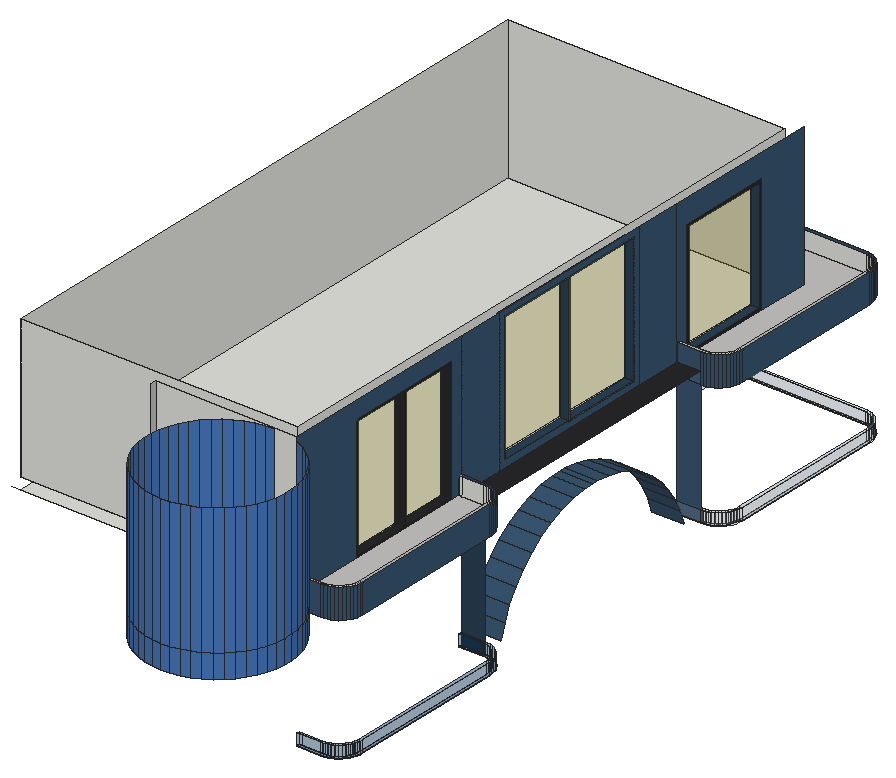
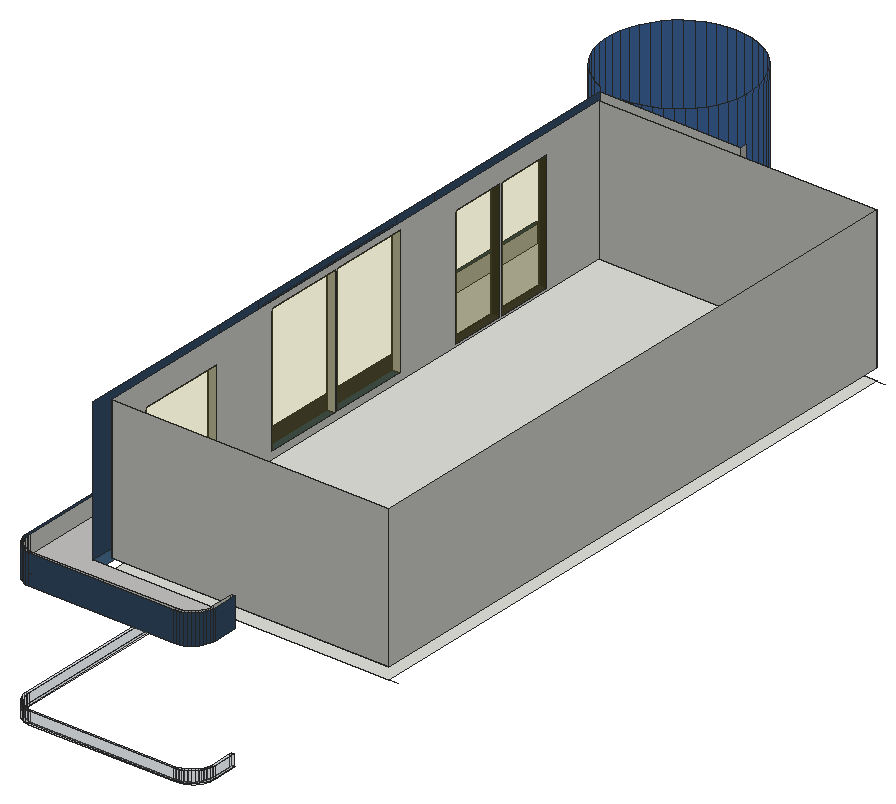
# SketchUp Ruby script. Lengths in inches.
U = 1.inch
M = Sketchup.active_model
def pt(a) = Geom::Point3d.new(a.map { |v| v * U })
def face(e, loops, mat)
  f = e.add_face(loops[0].map { |a| pt(a) })
  loops[1..].each { |l| e.add_face(l.map { |a| pt(a) }).erase! }
  f.material = f.back_material = mat if mat
  f
end
# faces: each face lists its corners as indices into pts; further lists are holes
def faces(e, pts, list, mat = nil) = list.each { |f| face(e, (f[0].is_a?(Array) ? f : [f]).map { |l| l.map { |i| pts[i] } }, mat) }
# xy, xz, yz: faces in a plane at the given z, y or x. An outline is a flat list of corners, or four numbers for a rectangle; further outlines are holes
def ring(l) = l.size == 4 ? [[l[0], l[1]], [l[2], l[1]], [l[2], l[3]], [l[0], l[3]]] : l.each_slice(2).to_a
def flat(e, list, mat, &to3) = list.each { |f| face(e, (f[0].is_a?(Array) ? f : [f]).map { |l| ring(l).map { |u, v| to3.(u, v) } }, mat) }
def xy(e, z, list, mat = nil) = flat(e, list, mat) { |x, y| [x, y, z] }
def xz(e, y, list, mat = nil) = flat(e, list, mat) { |x, z| [x, y, z] }
def yz(e, x, list, mat = nil) = flat(e, list, mat) { |y, z| [x, y, z] }
def lines(e, pts, list) = list.each { |a, b| e.add_line(pt(pts[a]), pt(pts[b])) }
# prism: a flat outline (further loops are holes) pulled along v
def prism(e, loops, v, mat = nil)
  f = face(e, loops, mat); d = Geom::Vector3d.new(v.map { |x| x * U })
  f.pushpull(f.normal.samedirection?(d) ? d.length : -d.length)
end
def box(e, o, s, mat = nil) = prism(e, [[o, [o[0] + s[0], o[1], o[2]], [o[0] + s[0], o[1] + s[1], o[2]], [o[0], o[1] + s[1], o[2]]]], [0, 0, s[2]], mat)
def at(x, y, z, deg = 0) = Geom::Transformation.translation(pt([x, y, z])) * Geom::Transformation.rotation(ORIGIN, Z_AXIS, deg.degrees)
def axes(o, x, y, z) = Geom::Transformation.new([*x, 0, *y, 0, *z, 0, *pt(o).to_a, 1])
def part(name) = M.definitions.add(name)
# library, detail: a bought-in or finely detailed component or shape, given as its bounding box
def library(name, o, s) = part(name).tap { |d| box(d.entities, o, s) }
def detail(e, o, s) = box(e.add_group.entities, o, s)
def put(e, d, t, mat = nil) = e.add_instance(d, t).tap { |i| i.material = mat if mat }
def group(e, t, mat = nil) = e.add_group.tap { |g| g.transformation = t; g.material = mat if mat }.entities
root = M.entities
M.materials.add("Carpet_01_1K").color = [196, 195, 193]
M.materials.add("Carpet_04_1K").color = [56, 85, 112]
M.materials.add("Carpet_04_1K1").color = [43, 65, 85]
M.materials.add("Glass_Basic_01").color = [186, 175, 28]
M.materials["Glass_Basic_01"].alpha = 0.25
M.materials.add("Glass_Basic_1").color = [0, 47, 91]
M.materials["Glass_Basic_1"].alpha = 0.25
M.materials.add("Glass_Basic_2").color = [161, 173, 186]
M.materials["Glass_Basic_2"].alpha = 0.25
M.materials.add("Glass_Mirror_01").color = [71, 118, 185]
M.materials.add("ThomThom - Buttons2").color = [40, 40, 43]
c1 = part("Group\#1")
prism(c1.entities,[[[0,206.04,0],[0,209.04,0],[24,209.04,0],[24.001,209.04,0],[27.133,208.835,0],[30.212,208.222,0],[33.184,207.213,0],[36,205.825,0],[38.61,204.081,0],[40.971,202.011,0],[43.04,199.65,0],[44.785,197.04,0],[46.173,194.224,0],[47.182,191.252,0],[47.795,188.173,0],[48,185.04,0],[48,24,0],[47.795,20.867,0],[47.182,17.788,0],[46.602,16.08,0],[46.173,14.816,0],[44.785,12,0],[43.04,9.39,0],[40.971,7.029,0],[38.61,4.96,0],[36,3.215,0],[33.184,1.827,0],[30.212,0.818,0],[27.133,0.205,0],[24,0,0],[0,0,0],[0,3,0],[3,3,0],[24,3,0],[26.741,3.18,0],[29.435,3.716,0],[32.036,4.599,0],[34.5,5.814,0],[36.784,7.34,0],[38.849,9.151,0],[40.66,11.216,0],[42.187,13.5,0],[43.401,15.964,0],[44.284,18.565,0],[44.82,21.259,0],[45,24,0],[45,185.04,0],[44.82,187.781,0],[44.284,190.475,0],[43.401,193.076,0],[42.187,195.54,0],[40.66,197.824,0],[38.849,199.889,0],[36.784,201.701,0],[34.5,203.227,0],[32.036,204.442,0],[29.435,205.325,0],[26.741,205.86,0],[24,206.04,0],[3,206.04,0]]],[0,0,12])
c2 = part("Group\#2")
prism(c2.entities,[[[147,3,0],[168,3,0],[170.74,3.18,0],[173.44,3.72,0],[176.04,4.6,0],[178.5,5.8125,0],[180.78,7.34,0],[182.85,9.15,0],[184.66,11.22,0],[186.1875,13.5,0],[187.4,15.96,0],[188.28,18.56,0],[188.82,21.26,0],[189,24,0],[189,184.94,0],[188.8125,187.78,0],[188.28,190.47,0],[187.4,193.07,0],[186.18,195.54,0],[184.66,197.82,0],[182.84,199.88,0],[180.78,201.7,0],[178.5,203.22,0],[176.03,204.4375,0],[173.43,205.32,0],[171.01,205.8,0],[24,205.8,0],[21.26,205.62,0],[18.56,205.08,0],[15.96,204.2,0],[13.5,202.99,0],[11.22,201.46,0],[9.15,199.65,0],[7.34,197.58,0],[5.8125,195.3,0],[4.6,192.84,0],[3.72,190.24,0],[3.18,187.54,0],[3,184.8,0],[3,163.8,0],[3,160.8,0],[0,160.8,0],[0,184.8,0],[0.21,187.93,0],[0.82,191.01,0],[1.83,193.98,0],[3.22,196.8,0],[4.96,199.41,0],[7.03,201.77,0],[9.39,203.84,0],[12,205.58,0],[14.82,206.97,0],[17.79,207.98,0],[20.87,208.59,0],[24,208.8,0],[171.31,208.8,0],[174.21,208.22,0],[177.18,207.21,0],[180,205.82,0],[182.61,204.08,0],[184.97,202.01,0],[187.04,199.65,0],[188.78,197.04,0],[190.17,194.22,0],[191.18,191.25,0],[191.79,188.17,0],[192,185.04,0],[192,24,0],[191.79,20.87,0],[191.18,17.79,0],[190.17,14.82,0],[188.78,12,0],[187.04,9.39,0],[184.97,7.03,0],[182.61,4.96,0],[180,3.22,0],[177.18,1.83,0],[174.21,0.82,0],[171.13,0.21,0],[168,0,0],[144,0,0],[144,3,0]]],[0,0,12])
xy(root,791.9,[[330.57,637.9,354.57,637.9,357.71,638.11,360.79,638.72,363.76,639.73,366.57,641.12,369.19,642.86,371.55,644.93,373.62,647.29,375.36,649.9,376.75,652.72,377.76,655.6875,378.37,658.77,378.57,661.9,378.57,822.94,378.37,826.07,377.76,829.15,376.75,832.125,375.36,834.94,373.62,837.55,371.55,839.91,369.19,841.98,366.57,843.73,363.76,845.11,360.79,846.12,357.88,846.7,210.57,846.7,207.44,846.5,204.36,845.88,201.39,844.875,198.57,843.49,195.96,841.74,193.6,839.67,191.53,837.3125,189.79,834.7,188.4,831.89,187.39,828.91,186.78,825.83,186.57,822.7,186.57,798.7,189.57,798.7,189.57,822.7,189.75,825.44,190.29,828.14,191.17,830.74,192.39,833.2,193.91,835.48,195.73,837.55,197.79,839.36,200.07,840.89,202.54,842.1,205.14,842.99,207.83,843.52,210.57,843.7,357.59,843.7,360.01,843.22,362.61,842.34,365.07,841.12,367.36,839.6,369.42,837.79,371.23,835.72,372.76,833.4375,373.97,830.97,374.85,828.375,375.39,825.68,375.57,822.84,375.57,661.9,375.4,659.16,374.86,656.47,373.98,653.86,372.76,651.4,371.24,649.12,369.42,647.05,367.36,645.24,365.07,643.71,362.61,642.5,360.01,641.62,357.32,641.08,354.57,640.9,330.57,640.9]])
xy(root,792,[[330.57,155.5,354.57,155.5,357.71,155.71,360.79,156.32,363.76,157.33,366.57,158.72,369.19,160.46,371.55,162.53,373.62,164.89,375.36,167.5,376.75,170.32,377.76,173.29,378.37,176.37,378.57,179.5,378.57,340.54,378.37,343.67,377.76,346.75,376.75,349.73,375.36,352.54,373.62,355.15,371.55,357.51,369.19,359.58,366.57,361.33,363.76,362.71,360.79,363.72,357.71,364.34,354.57,364.54,330.57,364.54,330.57,361.54,354.57,361.54,357.32,361.36,360.01,360.83,362.61,359.94,365.07,358.73,367.36,357.2,369.42,355.39,371.24,353.33,372.76,351.04,373.98,348.58,374.86,345.98,375.4,343.28,375.57,340.54,375.57,179.5,375.4,176.76,374.86,174.07,373.98,171.46,372.76,169,371.24,166.72,369.42,164.65,367.36,162.84,365.07,161.31,362.61,160.1,360.01,159.22,357.32,158.68,354.57,158.5,330.57,158.5]])
xy(root,891,[[321.57,652.9,330.57,742.9]])
xy(root,898,[[321.57,233.15,330.57,291.15],[321.57,293.15,330.57,349.15]],"ThomThom - Buttons2")
xy(root,918,[[39.57,167.5625,321.57,786.64]])
xy(root,918,[[330.57,155.5,330.57,364.54,354.57,364.54,357.71,364.34,360.79,363.72,363.76,362.71,366.57,361.33,369.19,359.58,371.55,357.51,373.62,355.15,375.36,352.54,376.75,349.73,377.76,346.75,378.37,343.67,378.57,340.54,378.57,179.5,378.37,176.37,377.76,173.29,376.75,170.32,375.36,167.5,373.62,164.89,371.55,162.53,369.19,160.46,366.57,158.72,363.76,157.33,360.79,156.32,357.71,155.71,354.57,155.5],[330.57,637.9,330.57,798.7,186.57,798.7,186.57,822.7,186.78,825.83,187.39,828.91,188.4,831.89,189.79,834.7,191.53,837.3125,193.6,839.67,195.96,841.74,198.57,843.49,201.39,844.875,204.36,845.88,207.44,846.5,210.57,846.7,357.88,846.7,360.79,846.12,363.76,845.11,366.57,843.73,369.19,841.98,371.55,839.91,373.62,837.55,375.36,834.94,376.75,832.125,377.76,829.15,378.37,826.07,378.57,822.94,378.57,661.9,378.37,658.77,377.76,655.6875,376.75,652.72,375.36,649.9,373.62,647.29,371.55,644.93,369.19,642.86,366.57,641.12,363.76,639.73,360.79,638.72,357.71,638.11,354.57,637.9]],"Carpet_04_1K")
xy(root,930,[[39.57,167.5625,321.57,786.64]])
xy(root,930,[[330.57,158.5,354.57,158.5,357.32,158.68,360.01,159.22,362.61,160.1,365.07,161.31,367.36,162.84,369.42,164.65,371.24,166.72,372.76,169,373.98,171.46,374.86,174.07,375.4,176.76,375.57,179.5,375.57,340.54,375.4,343.28,374.86,345.98,373.98,348.58,372.76,351.04,371.24,353.33,369.42,355.39,367.36,357.2,365.07,358.73,362.61,359.94,360.01,360.83,357.32,361.36,354.57,361.54,330.57,361.54],[330.57,640.9,354.57,640.9,357.32,641.08,360.01,641.62,362.61,642.5,365.07,643.71,367.36,645.24,369.42,647.05,371.24,649.12,372.76,651.4,373.98,653.86,374.86,656.47,375.4,659.16,375.57,661.9,375.57,822.84,375.39,825.68,374.85,828.375,373.97,830.97,372.76,833.4375,371.23,835.72,369.42,837.79,367.36,839.6,365.07,841.12,362.61,842.34,360.01,843.22,357.59,843.7,210.57,843.7,207.83,843.52,205.14,842.99,202.54,842.1,200.07,840.89,197.79,839.36,195.73,837.55,193.91,835.48,192.39,833.2,191.17,830.74,190.29,828.14,189.75,825.44,189.57,822.7,189.57,798.7,330.57,798.7]],"Carpet_01_1K")
xy(root,930,[[330.57,364.54,354.57,637.9]],"ThomThom - Buttons2")
xy(root,932,[[321.57,233.15,330.57,291.15],[321.57,293.15,330.57,349.15]],"ThomThom - Buttons2")
xy(root,933,[[321.57,652.9,330.57,742.9]],"Carpet_04_1K1")
xy(root,937,[[321.57,419.54,330.57,500.22],[321.57,502.22,330.57,582.9]],"Carpet_04_1K1")
xz(root,155.5,[[186.57,918,330.57,930],[186.57,930,330.57,1074]])
xz(root,155.5,[[330.57,918,354.57,948]],"Carpet_04_1K")
xz(root,158.5,[[330.57,930,333.57,948],[333.57,930,354.57,948]])
xz(root,167.5625,[[39.57,930,321.57,1074]])
xz(root,233.15,[[321.57,932,330.57,1054]],"ThomThom - Buttons2")
xz(root,291.15,[[321.57,932,330.57,1054]],"ThomThom - Buttons2")
xz(root,293.15,[[321.57,932,330.57,1054]],"ThomThom - Buttons2")
xz(root,349.15,[[321.57,932,330.57,1054]],"ThomThom - Buttons2")
xz(root,361.54,[[330.57,930,333.57,948],[333.57,930,354.57,948]])
xz(root,364.54,[[330.57,930,354.57,948]],"Carpet_04_1K")
xz(root,364.54,[[330.57,792,354.57,918]],"Carpet_04_1K1")
xz(root,419.54,[[321.57,937,330.57,1067]])
xz(root,500.22,[[321.57,937,330.57,1067]],"Carpet_04_1K1")
xz(root,502.22,[[321.57,937,330.57,1067]])
xz(root,582.9,[[321.57,937,330.57,1067]],"Carpet_04_1K1")
xz(root,637.9,[[330.57,791.9,354.57,918],[330.57,930,354.57,948]],"Carpet_04_1K")
xz(root,640.9,[[330.57,930,333.57,948],[333.57,930,354.57,948]])
xz(root,652.9,[[321.57,933,330.57,1047]])
xz(root,742.9,[[321.57,933,330.57,1047]],"Carpet_04_1K1")
xz(root,786.64,[[39.57,930,321.57,1074]])
xz(root,798.7,[[186.57,930,189.57,948]])
xz(root,843.7,[[210.57,930,357.59,948]])
xz(root,846.7,[[210.57,918,357.88,948]],"Carpet_04_1K")
yz(root,39.57,[[167.5625,930,786.64,1074]])
yz(root,186.57,[[149.51,918,155.5,930],[149.51,930,155.5,1074]],"Carpet_01_1K")
yz(root,186.57,[[798.7,918,822.7,948]],"Carpet_04_1K")
yz(root,189.57,[[798.7,930,801.7,948],[801.7,930,822.7,948]])
yz(root,236.92,[[77.22,918,86.26,942],[77.22,942,86.26,1074]],"Glass_Mirror_01")
yz(root,321.57,[[383.82,791.9375,384.21,794.33,384.27,794.54],[[167.5625,930,786.64,1074],[419.54,937,500.22,1067],[502.22,937,582.9,1067],[652.9,933,742.9,1047],[233.15,932,291.15,1054],[293.15,932,349.15,1054]]])
yz(root,321.57,[[233.15,932,291.15,1054],[293.15,932,349.15,1054],[652.9,933,742.9,1047],[419.54,937,500.22,1067],[502.22,937,582.9,1067]],"Glass_Basic_01")
yz(root,330.57,[[155.5,930,158.5,948],[361.54,930,364.54,948],[637.9,930,640.9,948]])
yz(root,330.57,[[158.5,930,231.15,930,231.15,1056,351.15,1056,351.15,930,361.54,930,361.54,948,364.54,948,364.54,1074,155.5,1074,155.5,948,158.5,948],[364.54,930,412.54,1074],[[412.54,930,589.9,1074],[418.54,936,583.9,1068]],[589.9,930,637.9,1074],[640.9,930,649.9,930,649.9,1050,745.9,1050,745.9,930,798.7,930,798.7,1074,637.9,1074,637.9,948,640.9,948],
  [[418.54,936,501.22,1068],[419.54,937,500.22,1067]],[[501.22,936,583.9,1068],[502.22,937,582.9,1067]]],"Carpet_04_1K")
yz(root,330.57,[[[231.15,930,351.15,1056],[233.15,932,233.15,1054,349.15,1054,349.15,932,293.15,932,293.15,1054,291.15,1054,291.15,932]],[[649.9,930,745.9,1050],[652.9,933,742.9,1047]]],"ThomThom - Buttons2")
yz(root,375.57,[[179.5,930,340.54,948],[661.9,930,822.84,948]])
yz(root,378.57,[[179.5,918,340.54,948],[661.9,918,822.94,948]],"Carpet_04_1K")
yz(root,380.64,[[77.22,918,86.26,942],[77.22,942,86.26,1074]],"Glass_Mirror_01")
p = [[321.57,388.88,810.1875],[354.57,388.88,810.1875],[354.57,384.48,795.78],[321.57,384.48,795.78],[321.57,616.9,799.9],[354.57,616.9,799.9],
  [354.57,611.99,814.15],[321.57,611.99,814.15],[321.57,395.06,823.9375],[354.57,395.06,823.9375],[354.57,605.34,827.67],[321.57,605.34,827.67],
  [321.57,402.9,836.8],[354.57,402.9,836.8],[354.57,597.04,840.25],[321.57,597.04,840.25],[321.57,412.3,848.58],[354.57,412.3,848.58],
  [354.57,587.23,851.68],[321.57,587.23,851.68],[321.57,423.1,859.09],[354.57,423.1,859.09],[354.57,576.06,861.8],[321.57,576.06,861.8],
  [321.57,435.13,868.16],[354.57,435.13,868.16],[354.57,563.71,870.44],[321.57,563.71,870.44],[321.57,448.21,875.66],[354.57,448.21,875.66],
  [354.57,550.38,877.47],[321.57,550.38,877.47],[321.57,462.12,881.45],[354.57,462.12,881.45],[354.57,536.27,882.77],[321.57,536.27,882.77],
  [321.57,476.65,885.46],[354.57,476.65,885.46],[354.57,521.61,886.25],[321.57,521.61,886.25],[321.57,491.5625,887.61],[354.57,491.5625,887.61],
  [354.57,506.63,887.88],[321.57,506.63,887.88],[321.57,501.22,887.78],[354.57,501.22,887.78],[308.78,9.74,918],[308.78,9.74,942],
  [299.76,10.31,942],[299.76,10.31,918],[317.8,10.31,918],[317.8,10.31,942],[290.875,12,942],[290.875,12,918],
  [326.6875,12,918],[326.6875,12,942],[282.28,14.79,942],[282.28,14.79,918],[335.29,14.79,918],[335.29,14.79,942],
  [274.09,18.64,942],[274.09,18.64,918],[343.47,18.64,918],[343.47,18.64,942],[266.46,23.49,942],[266.46,23.49,918],
  [351.1,23.49,918],[351.1,23.49,942],[259.49,29.25,942],[259.49,29.25,918],[358.07,29.25,918],[358.07,29.25,942],
  [253.3,35.84,942],[253.3,35.84,918],[364.26,35.84,918],[364.26,35.84,942],[247.99,43.16,942],[247.99,43.16,918],
  [369.57,43.16,918],[369.57,43.16,942],[243.63,51.08,942],[243.63,51.08,918],[373.93,51.08,918],[373.93,51.08,942],
  [240.3,59.49,942],[240.3,59.49,918],[377.26,59.49,918],[377.26,59.49,942],[238.06,68.25,942],[238.06,68.25,918],
  [379.51,68.25,918],[379.51,68.25,942],[236.92,77.22,942],[236.92,77.22,918],[380.64,77.22,918],[380.64,77.22,942],
  [236.92,86.26,918],[236.92,86.26,942],[238.06,95.23,942],[238.06,95.23,918],[379.51,95.23,918],[379.51,95.23,942],
  [380.64,86.26,942],[380.64,86.26,918],[240.3,103.99,942],[240.3,103.99,918],[377.26,103.99,918],[377.26,103.99,942],
  [243.63,112.39,942],[243.63,112.39,918],[373.93,112.39,918],[373.93,112.39,942],[247.99,120.32,942],[247.99,120.32,918],
  [369.57,120.32,918],[369.57,120.32,942],[253.3,127.63,942],[253.3,127.63,918],[364.26,127.63,918],[364.26,127.63,942],
  [259.49,134.22,942],[259.49,134.22,918],[358.07,134.22,918],[358.07,134.22,942],[266.46,139.99,942],[266.46,139.99,918],
  [351.1,139.99,918],[351.1,139.99,942],[274.09,144.83,942],[274.09,144.83,918],[343.47,144.83,918],[343.47,144.83,942],
  [282.28,148.68,942],[282.28,148.68,918],[335.29,148.68,918],[335.29,148.68,942],[290.875,151.48,942],[290.875,151.48,918],
  [299.76,153.17,942],[299.76,153.17,918],[308.78,153.74,942],[308.78,153.74,918],[357.71,155.71,918],[357.71,155.71,948],
  [354.57,155.5,948],[354.57,155.5,918],[360.79,156.32,918],[360.79,156.32,948],[363.76,157.33,918],[363.76,157.33,948],
  [366.57,158.72,918],[366.57,158.72,948],[369.19,160.46,918],[369.19,160.46,948],[371.55,162.53,918],[371.55,162.53,948],
  [373.62,164.89,918],[373.62,164.89,948],[375.36,167.5,918],[375.36,167.5,948],[376.75,170.32,918],[376.75,170.32,948],
  [377.76,173.29,918],[377.76,173.29,948],[378.37,176.37,918],[378.37,176.37,948],[378.57,179.5,918],[378.57,179.5,948],
  [378.37,343.67,918],[378.37,343.67,948],[378.57,340.54,948],[378.57,340.54,918],[377.76,346.75,918],[377.76,346.75,948],
  [376.75,349.73,918],[376.75,349.73,948],[375.36,352.54,918],[375.36,352.54,948],[373.62,355.15,918],[373.62,355.15,948],
  [371.55,357.51,918],[371.55,357.51,948],[369.19,359.58,918],[369.19,359.58,948],[366.57,361.33,918],[366.57,361.33,948],
  [363.76,362.71,918],[363.76,362.71,948],[360.79,363.72,918],[360.79,363.72,948],[357.71,364.34,918],[357.71,364.34,948],
  [354.57,364.54,918],[354.57,364.54,930],[354.57,364.54,948],[357.71,638.11,918],[357.71,638.11,948],[354.57,637.9,948],
  [354.57,637.9,930],[354.57,637.9,918],[360.79,638.72,918],[360.79,638.72,948],[363.76,639.73,918],[363.76,639.73,948],
  [366.57,641.12,918],[366.57,641.12,948],[369.19,642.86,918],[369.19,642.86,948],[371.55,644.93,918],[371.55,644.93,948],
  [373.62,647.29,918],[373.62,647.29,948],[375.36,649.9,918],[375.36,649.9,948],[376.75,652.72,918],[376.75,652.72,948],
  [377.76,655.6875,918],[377.76,655.6875,948],[378.37,658.77,918],[378.37,658.77,948],[378.57,661.9,918],[378.57,661.9,948],
  [186.57,822.7,918],[186.57,822.7,948],[186.78,825.83,948],[186.78,825.83,918],[378.37,826.07,918],[378.37,826.07,948],
  [378.57,822.94,948],[378.57,822.94,918],[187.39,828.91,948],[187.39,828.91,918],[377.76,829.15,918],[377.76,829.15,948],
  [188.4,831.89,948],[188.4,831.89,918],[376.75,832.125,918],[376.75,832.125,948],[189.79,834.7,948],[189.79,834.7,918],
  [375.36,834.94,918],[375.36,834.94,948],[191.53,837.3125,948],[191.53,837.3125,918],[373.62,837.55,918],[373.62,837.55,948],
  [193.6,839.67,948],[193.6,839.67,918],[371.55,839.91,918],[371.55,839.91,948],[195.96,841.74,948],[195.96,841.74,918],
  [369.19,841.98,918],[369.19,841.98,948],[198.57,843.49,948],[198.57,843.49,918],[366.57,843.73,918],[366.57,843.73,948],
  [201.39,844.875,948],[201.39,844.875,918],[363.76,845.11,918],[363.76,845.11,948],[204.36,845.88,948],[204.36,845.88,918],
  [360.79,846.12,918],[360.79,846.12,948],[207.44,846.5,948],[207.44,846.5,918],[357.88,846.7,930],[357.88,846.7,948],
  [357.88,846.7,918],[210.57,846.7,948],[210.57,846.7,918],[357.32,158.68,930],[354.57,158.5,930],[354.57,158.5,948],
  [357.32,158.68,948],[360.01,159.22,930],[360.01,159.22,948],[362.61,160.1,930],[362.61,160.1,948],[365.07,161.31,930],
  [365.07,161.31,948],[367.36,162.84,930],[367.36,162.84,948],[369.42,164.65,930],[369.42,164.65,948],[371.24,166.72,930],
  [371.24,166.72,948],[372.76,169,930],[372.76,169,948],[373.98,171.46,930],[373.98,171.46,948],[374.86,174.07,930],
  [374.86,174.07,948],[375.4,176.76,930],[375.4,176.76,948],[375.57,179.5,930],[375.57,179.5,948],[375.4,343.28,930],
  [375.57,340.54,930],[375.57,340.54,948],[375.4,343.28,948],[374.86,345.98,930],[374.86,345.98,948],[373.98,348.58,930],
  [373.98,348.58,948],[372.76,351.04,930],[372.76,351.04,948],[371.24,353.33,930],[371.24,353.33,948],[369.42,355.39,930],
  [369.42,355.39,948],[367.36,357.2,930],[367.36,357.2,948],[365.07,358.73,930],[365.07,358.73,948],[362.61,359.94,930],
  [362.61,359.94,948],[360.01,360.83,930],[360.01,360.83,948],[357.32,361.36,930],[357.32,361.36,948],[354.57,361.54,930],
  [354.57,361.54,948],[357.32,641.08,930],[354.57,640.9,930],[354.57,640.9,948],[357.32,641.08,948],[360.01,641.62,930],
  [360.01,641.62,948],[362.61,642.5,930],[362.61,642.5,948],[365.07,643.71,930],[365.07,643.71,948],[367.36,645.24,930],
  [367.36,645.24,948],[369.42,647.05,930],[369.42,647.05,948],[371.24,649.12,930],[371.24,649.12,948],[372.76,651.4,930],
  [372.76,651.4,948],[373.98,653.86,930],[373.98,653.86,948],[374.86,656.47,930],[374.86,656.47,948],[375.4,659.16,930],
  [375.4,659.16,948],[375.57,661.9,930],[375.57,661.9,948],[189.57,822.7,930],[189.75,825.44,930],[189.75,825.44,948],
  [189.57,822.7,948],[375.39,825.68,930],[375.57,822.84,930],[375.57,822.84,948],[375.39,825.68,948],[190.29,828.14,930],
  [190.29,828.14,948],[374.85,828.375,930],[374.85,828.375,948],[191.17,830.74,930],[191.17,830.74,948],[373.97,830.97,930],
  [373.97,830.97,948],[192.39,833.2,930],[192.39,833.2,948],[372.76,833.4375,930],[372.76,833.4375,948],[193.91,835.48,930],
  [193.91,835.48,948],[371.23,835.72,930],[371.23,835.72,948],[195.73,837.55,930],[195.73,837.55,948],[369.42,837.79,930],
  [369.42,837.79,948],[197.79,839.36,930],[197.79,839.36,948],[367.36,839.6,930],[367.36,839.6,948],[200.07,840.89,930],
  [200.07,840.89,948],[365.07,841.12,930],[365.07,841.12,948],[202.54,842.1,930],[202.54,842.1,948],[362.61,842.34,930],
  [362.61,842.34,948],[205.14,842.99,930],[205.14,842.99,948],[360.01,843.22,930],[360.01,843.22,948],[207.83,843.52,930],
  [207.83,843.52,948],[357.59,843.7,930],[357.59,843.7,948],[210.57,843.7,930],[210.57,843.7,948],[299.76,10.31,1074],
  [308.78,9.74,1074],[317.8,10.31,1074],[290.875,12,1074],[326.6875,12,1074],[282.28,14.79,1074],[335.29,14.79,1074],
  [274.09,18.64,1074],[343.47,18.64,1074],[266.46,23.49,1074],[351.1,23.49,1074],[259.49,29.25,1074],[358.07,29.25,1074],
  [253.3,35.84,1074],[364.26,35.84,1074],[247.99,43.16,1074],[369.57,43.16,1074],[243.63,51.08,1074],[373.93,51.08,1074],
  [240.3,59.49,1074],[377.26,59.49,1074],[238.06,68.25,1074],[379.51,68.25,1074],[236.92,77.22,1074],[380.64,77.22,1074],
  [238.06,95.23,1074],[236.92,86.26,1074],[380.64,86.26,1074],[379.51,95.23,1074],[240.3,103.99,1074],[377.26,103.99,1074],
  [243.63,112.39,1074],[373.93,112.39,1074],[247.99,120.32,1074],[369.57,120.32,1074],[253.3,127.63,1074],[364.26,127.63,1074],
  [259.49,134.22,1074],[358.07,134.22,1074],[266.46,139.99,1074],[351.1,139.99,1074],[274.09,144.83,1074],[343.47,144.83,1074],
  [282.28,148.68,1074],[335.29,148.68,1074],[290.875,151.48,1074],[299.76,153.17,1074],[308.78,153.74,1074],[321.57,786.64,918],
  [330.57,786.64,918],[39.57,786.64,918],[30.57,786.64,918],[39.57,167.5625,918],[30.57,167.5625,918],[321.57,167.5625,918],
  [330.57,167.5625,918],[357.71,846.74,930],[354.57,846.94,930],[330.57,150.21,918],[330.57,150.21,942]]
faces(root,p,[[0,1,2,3],[4,5,6,7],[8,9,1,0],[7,6,10,11],[12,13,9,8],[11,10,14,15],[16,17,13,12],[15,14,18,19],
  [20,21,17,16],[19,18,22,23],[24,25,21,20],[23,22,26,27],[28,29,25,24],[27,26,30,31],[32,33,29,28],[31,30,34,35],
  [36,37,33,32],[35,34,38,39],[40,41,37,36],[39,38,42,43],[44,45,41,40],[43,42,45,44],[142,143,144,145],[146,147,143,142],
  [148,149,147,146],[150,151,149,148],[152,153,151,150],[154,155,153,152],[156,157,155,154],[158,159,157,156],[160,161,159,158],[162,163,161,160],
  [164,165,163,162],[166,167,165,164],[168,169,170,171],[172,173,169,168],[174,175,173,172],[176,177,175,174],[178,179,177,176],[180,181,179,178],
  [182,183,181,180],[184,185,183,182],[186,187,185,184],[188,189,187,186],[190,191,189,188],[192,193,194,191,190],[195,196,197,198,199],[200,201,196,195],
  [202,203,201,200],[204,205,203,202],[206,207,205,204],[208,209,207,206],[210,211,209,208],[212,213,211,210],[214,215,213,212],[216,217,215,214],
  [218,219,217,216],[220,221,219,218],[222,223,224,225],[226,227,228,229],[225,224,230,231],[232,233,227,226],[231,230,234,235],[236,237,233,232],
  [235,234,238,239],[240,241,237,236],[239,238,242,243],[244,245,241,240],[243,242,246,247],[248,249,245,244],[247,246,250,251],[252,253,249,248],
  [251,250,254,255],[256,257,253,252],[255,254,258,259],[260,261,257,256],[259,258,262,263],[264,265,261,260],[263,262,266,267],[268,269,265,264,270],
  [267,266,271,272]],"Carpet_04_1K")
faces(root,p,[[46,47,48,49],[50,51,47,46],[49,48,52,53],[54,55,51,50],[53,52,56,57],[58,59,55,54],[57,56,60,61],[62,63,59,58],
  [61,60,64,65],[66,67,63,62],[65,64,68,69],[70,71,67,66],[69,68,72,73],[74,75,71,70],[73,72,76,77],[78,79,75,74],
  [77,76,80,81],[82,83,79,78],[81,80,84,85],[86,87,83,82],[85,84,88,89],[90,91,87,86],[89,88,92,93],[94,95,91,90],
  [96,97,98,99],[100,101,102,103],[99,98,104,105],[106,107,101,100],[105,104,108,109],[110,111,107,106],[109,108,112,113],[114,115,111,110],
  [113,112,116,117],[118,119,115,114],[117,116,120,121],[122,123,119,118],[121,120,124,125],[126,127,123,122],[125,124,128,129],[130,131,127,126],
  [129,128,132,133],[134,135,131,130],[133,132,136,137],[137,136,138,139],[139,138,140,141],[401,48,47,402],[402,47,51,403],[404,52,48,401],
  [403,51,55,405],[406,56,52,404],[405,55,59,407],[408,60,56,406],[407,59,63,409],[410,64,60,408],[409,63,67,411],[412,68,64,410],
  [411,67,71,413],[414,72,68,412],[413,71,75,415],[416,76,72,414],[415,75,79,417],[418,80,76,416],[417,79,83,419],[420,84,80,418],
  [419,83,87,421],[422,88,84,420],[421,87,91,423],[424,92,88,422],[423,91,95,425],[426,98,97,427],[428,102,101,429],[430,104,98,426],
  [429,101,107,431],[432,108,104,430],[431,107,111,433],[434,112,108,432],[433,111,115,435],[436,116,112,434],[435,115,119,437],[438,120,116,436],
  [437,119,123,439],[440,124,120,438],[439,123,127,441],[442,128,124,440],[441,127,131,443],[444,132,128,442],[443,131,135,445],[446,136,132,444],
  [447,138,136,446],[448,140,138,447]],"Glass_Mirror_01")
faces(root,p,[[273,274,275,276],[277,273,276,278],[279,277,278,280],[281,279,280,282],[283,281,282,284],[285,283,284,286],[287,285,286,288],[289,287,288,290],
  [291,289,290,292],[293,291,292,294],[295,293,294,296],[297,295,296,298],[299,300,301,302],[303,299,302,304],[305,303,304,306],[307,305,306,308],
  [309,307,308,310],[311,309,310,312],[313,311,312,314],[315,313,314,316],[317,315,316,318],[319,317,318,320],[321,319,320,322],[323,321,322,324],
  [325,326,327,328],[329,325,328,330],[331,329,330,332],[333,331,332,334],[335,333,334,336],[337,335,336,338],[339,337,338,340],[341,339,340,342],
  [343,341,342,344],[345,343,344,346],[347,345,346,348],[349,347,348,350],[351,352,353,354],[355,356,357,358],[352,359,360,353],[361,355,358,362],
  [359,363,364,360],[365,361,362,366],[363,367,368,364],[369,365,366,370],[367,371,372,368],[373,369,370,374],[371,375,376,372],[377,373,374,378],
  [375,379,380,376],[381,377,378,382],[379,383,384,380],[385,381,382,386],[383,387,388,384],[389,385,386,390],[387,391,392,388],[393,389,390,394],
  [391,395,396,392],[397,393,394,398],[395,399,400,396]])
lines(root,p,[[449,450],[451,452],[453,454],[455,456],[457,458],[268,457],[134,459],[135,460]])
put(root,c1,at(330.57,155.5,792),"Glass_Basic_1")
put(root,c2,at(186.57,637.9,792),"Glass_Basic_2")
